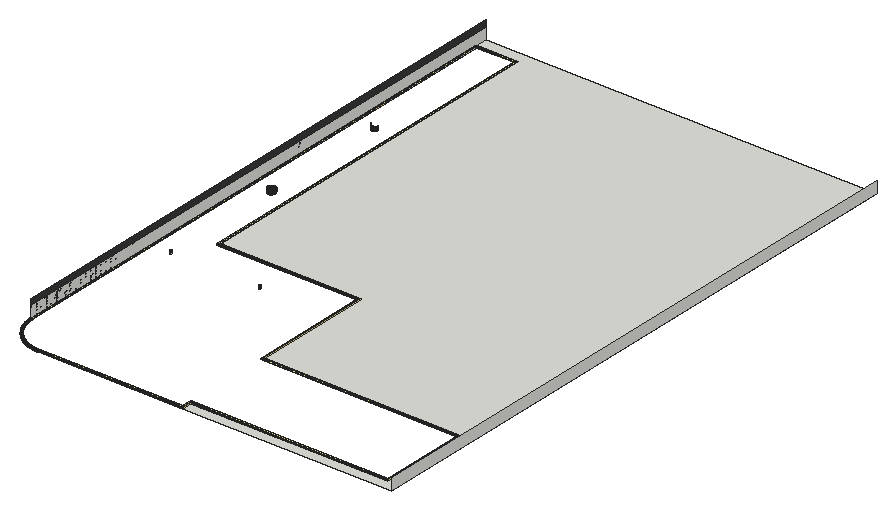
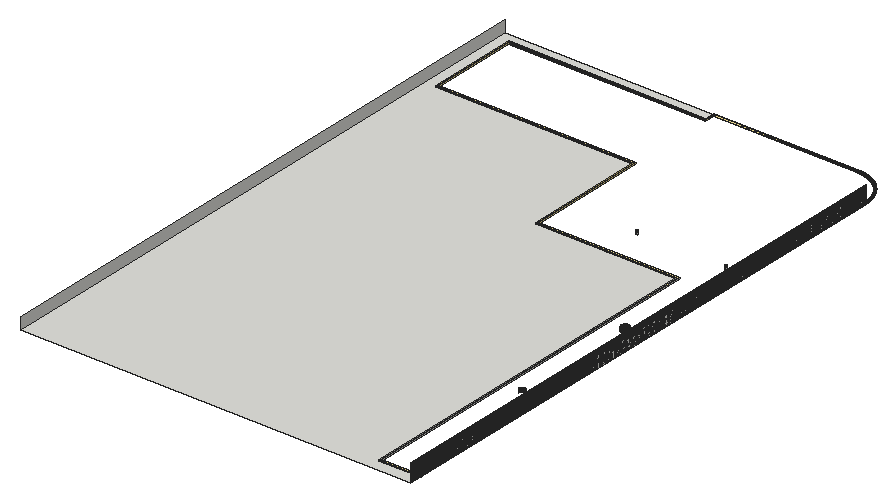
# SketchUp Ruby script. Lengths in inches.
U = 1.inch
M = Sketchup.active_model
def pt(a) = Geom::Point3d.new(a.map { |v| v * U })
def face(e, loops, mat)
  f = e.add_face(loops[0].map { |a| pt(a) })
  loops[1..].each { |l| e.add_face(l.map { |a| pt(a) }).erase! }
  f.material = f.back_material = mat if mat
  f
end
# faces: each face lists its corners as indices into pts; further lists are holes
def faces(e, pts, list, mat = nil) = list.each { |f| face(e, (f[0].is_a?(Array) ? f : [f]).map { |l| l.map { |i| pts[i] } }, mat) }
# xy, xz, yz: faces in a plane at the given z, y or x. An outline is a flat list of corners, or four numbers for a rectangle; further outlines are holes
def ring(l) = l.size == 4 ? [[l[0], l[1]], [l[2], l[1]], [l[2], l[3]], [l[0], l[3]]] : l.each_slice(2).to_a
def flat(e, list, mat, &to3) = list.each { |f| face(e, (f[0].is_a?(Array) ? f : [f]).map { |l| ring(l).map { |u, v| to3.(u, v) } }, mat) }
def xy(e, z, list, mat = nil) = flat(e, list, mat) { |x, y| [x, y, z] }
def xz(e, y, list, mat = nil) = flat(e, list, mat) { |x, z| [x, y, z] }
def yz(e, x, list, mat = nil) = flat(e, list, mat) { |y, z| [x, y, z] }
def lines(e, pts, list) = list.each { |a, b| e.add_line(pt(pts[a]), pt(pts[b])) }
# prism: a flat outline (further loops are holes) pulled along v
def prism(e, loops, v, mat = nil)
  f = face(e, loops, mat); d = Geom::Vector3d.new(v.map { |x| x * U })
  f.pushpull(f.normal.samedirection?(d) ? d.length : -d.length)
end
def box(e, o, s, mat = nil) = prism(e, [[o, [o[0] + s[0], o[1], o[2]], [o[0] + s[0], o[1] + s[1], o[2]], [o[0], o[1] + s[1], o[2]]]], [0, 0, s[2]], mat)
def at(x, y, z, deg = 0) = Geom::Transformation.translation(pt([x, y, z])) * Geom::Transformation.rotation(ORIGIN, Z_AXIS, deg.degrees)
def axes(o, x, y, z) = Geom::Transformation.new([*x, 0, *y, 0, *z, 0, *pt(o).to_a, 1])
def part(name) = M.definitions.add(name)
# library, detail: a bought-in or finely detailed component or shape, given as its bounding box
def library(name, o, s) = part(name).tap { |d| box(d.entities, o, s) }
def detail(e, o, s) = box(e.add_group.entities, o, s)
def put(e, d, t, mat = nil) = e.add_instance(d, t).tap { |i| i.material = mat if mat }
def group(e, t, mat = nil) = e.add_group.tap { |g| g.transformation = t; g.material = mat if mat }.entities
root = M.entities
M.materials.add("1496 AP 8293 CARBON COPY").color = [58, 58, 58]
M.materials.add("False Ceiling Light").color = [251, 231, 149]
xy(root,129,[[158,85,158,93,314,93,314,165,158,165,158,261,47,261,47,555,14,555,14,564,323,564,323,85]])
xz(root,232.5,[[30.34,129,30.42,132],[30.42,129,30.5,132],[30.5,129,30.58,132],[30.58,129,30.66,132],[100.84,129,100.92,132],
  [100.92,129,101,132],[101,129,101.08,132],[101.08,129,101.16,132]])
xz(root,259.5,[[45.5,129,156.5,129.5]])
xz(root,261,[[47,129,158,129.5]])
xz(root,329,[[30.34,129,30.42,132],[30.42,129,30.5,132],[30.5,129,30.58,132],[30.58,129,30.66,132]])
xz(root,335,[[30.34,129,30.42,132],[30.42,129,30.5,132],[30.5,129,30.58,132],[30.58,129,30.66,132]])
xz(root,431.5,[[30.34,129,30.42,132],[30.42,129,30.5,132],[30.5,129,30.58,132],[30.58,129,30.66,132]])
yz(root,14,[[555,129,555,129.5,115,129.5,115,138,564,138,564,129]])
yz(root,14,[[115,129,564,143]],"1496 AP 8293 CARBON COPY")
yz(root,15.5,[[115,129,553.5,129.5]])
yz(root,27.5,[[331.84,129,331.92,132],[331.92,129,332,132],[332,129,332.08,132],[332.08,129,332.16,132]])
yz(root,33.5,[[331.84,129,331.92,132],[331.92,129,332,132],[332,129,332.08,132],[332.08,129,332.16,132]])
yz(root,45.5,[[259.5,129,553.5,129.5]])
yz(root,47,[[261,129,555,129.5]])
yz(root,323,[[85,129,564,138]])
p = [[30.97,232.46,129],[31.05,232.45,129],[31.05,232.45,132],[30.97,232.46,132],[30.03,232.46,129],[30.11,232.47,129],
  [30.11,232.47,132],[30.03,232.46,132],[30.1875,232.48,129],[30.1875,232.48,132],[30.26,232.49,129],[30.26,232.49,132],
  [30.34,232.5,129],[30.34,232.5,132],[30.74,232.49,129],[30.8125,232.48,129],[30.8125,232.48,132],[30.74,232.49,132],
  [30.66,232.5,129],[30.66,232.5,132],[30.89,232.47,129],[30.89,232.47,132],[100.53,232.46,129],[100.61,232.47,129],
  [100.61,232.47,132],[100.53,232.46,132],[100.6875,232.48,129],[100.6875,232.48,132],[100.76,232.49,129],[100.76,232.49,132],
  [100.84,232.5,129],[100.84,232.5,132],[101.24,232.49,129],[101.3125,232.48,129],[101.3125,232.48,132],[101.24,232.49,132],
  [101.16,232.5,129],[101.16,232.5,132],[101.39,232.47,129],[101.39,232.47,132],[101.47,232.46,129],[101.47,232.46,132],
  [30.11,329.03,129],[30.03,329.04,129],[30.03,329.04,132],[30.11,329.03,132],[29.95,329.05,129],[29.95,329.05,132],
  [30.1875,329.02,129],[30.1875,329.02,132],[30.26,329.01,129],[30.26,329.01,132],[30.34,329,129],[30.34,329,132],
  [30.74,329.01,129],[30.66,329,129],[30.66,329,132],[30.74,329.01,132],[30.8125,329.02,129],[30.8125,329.02,132],
  [30.89,329.03,129],[30.89,329.03,132],[30.97,329.04,129],[30.97,329.04,132],[31.05,329.05,129],[31.05,329.05,132],
  [29.57,329.15,129],[29.5,329.17,129],[29.5,329.17,132],[29.57,329.15,132],[29.72,329.1,129],[29.65,329.125,129],
  [29.65,329.125,132],[29.72,329.1,132],[29.8,329.08,129],[29.8,329.08,132],[29.875,329.07,129],[29.875,329.07,132],
  [31.125,329.07,129],[31.125,329.07,132],[31.2,329.08,129],[31.2,329.08,132],[31.28,329.1,129],[31.28,329.1,132],
  [31.35,329.125,129],[31.35,329.125,132],[31.43,329.15,129],[31.43,329.15,132],[31.5,329.17,129],[31.5,329.17,132],
  [29.35,329.23,129],[29.28,329.26,129],[29.28,329.26,132],[29.35,329.23,132],[29.42,329.2,129],[29.42,329.2,132],
  [31.58,329.2,129],[31.58,329.2,132],[31.65,329.23,129],[31.65,329.23,132],[31.72,329.26,129],[31.72,329.26,132],
  [29.21,329.29,129],[29.14,329.33,129],[29.14,329.33,132],[29.21,329.29,132],[29.07,329.36,129],[29.07,329.36,132],
  [31.79,329.29,129],[31.79,329.29,132],[31.86,329.33,129],[31.86,329.33,132],[31.93,329.36,129],[31.93,329.36,132],
  [29,329.4,129],[28.93,329.44,129],[28.93,329.44,132],[29,329.4,132],[28.87,329.48,129],[28.87,329.48,132],
  [32,329.4,129],[32,329.4,132],[32.07,329.44,129],[32.07,329.44,132],[32.13,329.48,129],[32.13,329.48,132],
  [28.8,329.53,129],[28.74,329.57,129],[28.74,329.57,132],[28.8,329.53,132],[32.2,329.53,129],[32.2,329.53,132],
  [32.26,329.57,129],[32.26,329.57,132],[28.67,329.62,129],[28.61,329.67,129],[28.61,329.67,132],[28.67,329.62,132],
  [32.33,329.62,129],[32.33,329.62,132],[32.39,329.67,129],[32.39,329.67,132],[28.55,329.72,129],[28.49,329.77,129],
  [28.49,329.77,132],[28.55,329.72,132],[32.45,329.72,129],[32.45,329.72,132],[32.51,329.77,129],[32.51,329.77,132],
  [28.43,329.82,129],[28.43,329.82,132],[28.38,329.88,129],[28.38,329.88,132],[32.57,329.82,129],[32.57,329.82,132],
  [32.62,329.88,129],[32.62,329.88,132],[28.32,329.93,129],[28.32,329.93,132],[28.27,329.99,129],[28.27,329.99,132],
  [32.68,329.93,129],[32.68,329.93,132],[32.73,329.99,129],[32.73,329.99,132],[28.22,330.05,129],[28.22,330.05,132],
  [32.78,330.05,129],[32.78,330.05,132],[28.17,330.11,129],[28.12,330.17,129],[28.12,330.17,132],[28.17,330.11,132],
  [32.83,330.11,129],[32.83,330.11,132],[32.88,330.17,129],[32.88,330.17,132],[28.07,330.24,129],[28.03,330.3,129],
  [28.03,330.3,132],[28.07,330.24,132],[32.93,330.24,129],[32.93,330.24,132],[32.97,330.3,129],[32.97,330.3,132],
  [27.98,330.37,129],[27.98,330.37,132],[33.02,330.37,129],[33.02,330.37,132],[27.94,330.43,129],[27.94,330.43,132],
  [27.9,330.5,129],[27.9,330.5,132],[33.06,330.43,129],[33.06,330.43,132],[33.1,330.5,129],[33.1,330.5,132],
  [27.86,330.57,129],[27.86,330.57,132],[33.14,330.57,129],[33.14,330.57,132],[27.83,330.64,129],[27.83,330.64,132],
  [27.79,330.71,129],[27.79,330.71,132],[33.17,330.64,129],[33.17,330.64,132],[33.21,330.71,129],[33.21,330.71,132],
  [27.76,330.78,129],[27.76,330.78,132],[33.24,330.78,129],[33.24,330.78,132],[27.73,330.85,129],[27.73,330.85,132],
  [33.27,330.85,129],[33.27,330.85,132],[27.7,330.92,129],[27.7,330.92,132],[27.67,331,129],[27.67,331,132],
  [33.3,330.92,129],[33.3,330.92,132],[33.33,331,129],[33.33,331,132],[27.65,331.07,129],[27.65,331.07,132],
  [33.35,331.07,129],[33.35,331.07,132],[27.625,331.15,129],[27.625,331.15,132],[27.6,331.22,129],[27.6,331.22,132],
  [33.375,331.15,129],[33.375,331.15,132],[33.4,331.22,129],[33.4,331.22,132],[27.58,331.3,129],[27.58,331.3,132],
  [33.42,331.3,129],[33.42,331.3,132],[27.57,331.375,129],[27.57,331.375,132],[33.43,331.375,129],[33.43,331.375,132],
  [27.55,331.45,129],[27.55,331.45,132],[33.45,331.45,129],[33.45,331.45,132],[27.54,331.53,129],[27.54,331.53,132],
  [27.53,331.61,129],[27.53,331.61,132],[33.46,331.53,129],[33.46,331.53,132],[33.47,331.61,129],[33.47,331.61,132],
  [27.52,331.6875,129],[27.52,331.6875,132],[33.48,331.6875,129],[33.48,331.6875,132],[27.51,331.76,129],[27.51,331.76,132],
  [33.49,331.76,129],[33.49,331.76,132],[27.5,331.84,129],[27.5,331.84,132],[33.5,331.84,129],[33.5,331.84,132],
  [27.5,332.16,129],[27.51,332.24,129],[27.51,332.24,132],[27.5,332.16,132],[27.52,332.3125,129],[27.52,332.3125,132],
  [33.49,332.24,129],[33.5,332.16,129],[33.5,332.16,132],[33.49,332.24,132],[33.48,332.3125,129],[33.48,332.3125,132],
  [27.53,332.39,129],[27.53,332.39,132],[33.47,332.39,129],[33.47,332.39,132],[27.54,332.47,129],[27.54,332.47,132],
  [33.46,332.47,129],[33.46,332.47,132],[27.55,332.55,129],[27.55,332.55,132],[27.57,332.625,129],[27.57,332.625,132],
  [33.45,332.55,129],[33.45,332.55,132],[33.43,332.625,129],[33.43,332.625,132],[27.58,332.7,129],[27.58,332.7,132],
  [33.42,332.7,129],[33.42,332.7,132],[27.6,332.78,129],[27.6,332.78,132],[33.4,332.78,129],[33.4,332.78,132],
  [27.625,332.85,129],[27.625,332.85,132],[33.375,332.85,129],[33.375,332.85,132],[27.65,332.93,129],[27.65,332.93,132],
  [27.67,333,129],[27.67,333,132],[33.33,333,129],[33.35,332.93,129],[33.35,332.93,132],[33.33,333,132],
  [27.7,333.08,129],[27.7,333.08,132],[33.3,333.08,129],[33.3,333.08,132],[27.73,333.15,129],[27.73,333.15,132],
  [27.76,333.22,129],[27.76,333.22,132],[33.24,333.22,129],[33.27,333.15,129],[33.27,333.15,132],[33.24,333.22,132],
  [27.79,333.29,129],[27.79,333.29,132],[33.21,333.29,129],[33.21,333.29,132],[27.83,333.36,129],[27.83,333.36,132],
  [33.17,333.36,129],[33.17,333.36,132],[27.86,333.43,129],[27.86,333.43,132],[27.9,333.5,129],[27.9,333.5,132],
  [33.14,333.43,129],[33.14,333.43,132],[33.1,333.5,129],[33.1,333.5,132],[27.94,333.57,129],[27.94,333.57,132],
  [33.06,333.57,129],[33.06,333.57,132],[27.98,333.63,129],[27.98,333.63,132],[28.03,333.7,129],[28.03,333.7,132],
  [33.02,333.63,129],[33.02,333.63,132],[32.97,333.7,129],[32.97,333.7,132],[28.07,333.76,129],[28.07,333.76,132],
  [32.93,333.76,129],[32.93,333.76,132],[28.12,333.83,129],[28.12,333.83,132],[28.17,333.89,129],[28.17,333.89,132],
  [32.83,333.89,129],[32.88,333.83,129],[32.88,333.83,132],[32.83,333.89,132],[28.22,333.95,129],[28.22,333.95,132],
  [28.27,334.01,129],[28.27,334.01,132],[32.73,334.01,129],[32.78,333.95,129],[32.78,333.95,132],[32.73,334.01,132],
  [28.32,334.07,129],[28.32,334.07,132],[32.68,334.07,129],[32.68,334.07,132],[28.38,334.12,129],[28.38,334.12,132],
  [28.43,334.18,129],[28.43,334.18,132],[32.62,334.12,129],[32.62,334.12,132],[32.57,334.18,129],[32.57,334.18,132],
  [28.49,334.23,129],[28.49,334.23,132],[28.55,334.28,129],[28.55,334.28,132],[32.45,334.28,129],[32.51,334.23,129],
  [32.51,334.23,132],[32.45,334.28,132],[28.61,334.33,129],[28.61,334.33,132],[28.67,334.38,129],[28.67,334.38,132],
  [32.33,334.38,129],[32.39,334.33,129],[32.39,334.33,132],[32.33,334.38,132],[28.74,334.43,129],[28.74,334.43,132],
  [28.8,334.47,129],[28.8,334.47,132],[32.2,334.47,129],[32.26,334.43,129],[32.26,334.43,132],[32.2,334.47,132],
  [28.87,334.52,129],[28.87,334.52,132],[28.93,334.56,129],[28.93,334.56,132],[32.13,334.52,129],[32.13,334.52,132],
  [32.07,334.56,129],[32.07,334.56,132],[29,334.6,129],[29,334.6,132],[29.07,334.64,129],[29.07,334.64,132],
  [29.14,334.67,129],[29.14,334.67,132],[31.93,334.64,129],[32,334.6,129],[32,334.6,132],[31.93,334.64,132],
  [31.86,334.67,129],[31.86,334.67,132],[29.21,334.71,129],[29.21,334.71,132],[29.28,334.74,129],[29.28,334.74,132],
  [29.35,334.77,129],[29.35,334.77,132],[31.65,334.77,129],[31.72,334.74,129],[31.72,334.74,132],[31.65,334.77,132],
  [31.79,334.71,129],[31.79,334.71,132],[29.42,334.8,129],[29.42,334.8,132],[29.5,334.83,129],[29.5,334.83,132],
  [29.57,334.85,129],[29.57,334.85,132],[31.43,334.85,129],[31.5,334.83,129],[31.5,334.83,132],[31.43,334.85,132],
  [31.58,334.8,129],[31.58,334.8,132],[29.65,334.875,129],[29.65,334.875,132],[29.72,334.9,129],[29.72,334.9,132],
  [29.8,334.92,129],[29.8,334.92,132],[29.875,334.93,129],[29.875,334.93,132],[29.95,334.95,129],[29.95,334.95,132],
  [30.03,334.96,129],[30.03,334.96,132],[31.05,334.95,129],[31.125,334.93,129],[31.125,334.93,132],[31.05,334.95,132],
  [30.97,334.96,129],[30.97,334.96,132],[31.2,334.92,129],[31.2,334.92,132],[31.28,334.9,129],[31.28,334.9,132],
  [31.35,334.875,129],[31.35,334.875,132],[30.11,334.97,129],[30.11,334.97,132],[30.1875,334.98,129],[30.1875,334.98,132],
  [30.26,334.99,129],[30.26,334.99,132],[30.34,335,129],[30.34,335,132],[30.74,334.99,129],[30.8125,334.98,129],
  [30.8125,334.98,132],[30.74,334.99,132],[30.66,335,129],[30.66,335,132],[30.89,334.97,129],[30.89,334.97,132],
  [30.11,431.53,129],[30.03,431.54,129],[30.03,431.54,132],[30.11,431.53,132],[29.95,431.55,129],[29.95,431.55,132],
  [30.1875,431.52,129],[30.1875,431.52,132],[30.26,431.51,129],[30.26,431.51,132],[30.34,431.5,129],[30.34,431.5,132],
  [30.74,431.51,129],[30.66,431.5,129],[30.66,431.5,132],[30.74,431.51,132],[30.8125,431.52,129],[30.8125,431.52,132],
  [30.89,431.53,129],[30.89,431.53,132],[30.97,431.54,129],[30.97,431.54,132],[31.05,431.55,129],[31.05,431.55,132],
  [29.57,431.65,129],[29.5,431.67,129],[29.5,431.67,132],[29.57,431.65,132],[29.72,431.6,129],[29.65,431.625,129],
  [29.65,431.625,132],[29.72,431.6,132],[29.8,431.58,129],[29.8,431.58,132],[29.875,431.57,129],[29.875,431.57,132],
  [31.125,431.57,129],[31.125,431.57,132],[31.2,431.58,129],[31.2,431.58,132],[31.28,431.6,129],[31.28,431.6,132],
  [31.35,431.625,129],[31.35,431.625,132],[31.43,431.65,129],[31.43,431.65,132],[31.5,431.67,129],[31.5,431.67,132],
  [29.35,431.73,129],[29.28,431.76,129],[29.28,431.76,132],[29.35,431.73,132],[29.42,431.7,129],[29.42,431.7,132],
  [31.58,431.7,129],[31.58,431.7,132],[31.65,431.73,129],[31.65,431.73,132],[31.72,431.76,129],[31.72,431.76,132],
  [29.21,431.79,129],[29.14,431.83,129],[29.14,431.83,132],[29.21,431.79,132],[29.07,431.86,129],[29.07,431.86,132],
  [31.79,431.79,129],[31.79,431.79,132],[31.86,431.83,129],[31.86,431.83,132],[31.93,431.86,129],[31.93,431.86,132],
  [29,431.9,129],[28.93,431.94,129],[28.93,431.94,132],[29,431.9,132],[28.87,431.98,129],[28.87,431.98,132],
  [32,431.9,129],[32,431.9,132],[32.07,431.94,129],[32.07,431.94,132],[32.13,431.98,129],[32.13,431.98,132],
  [28.8,432.03,129],[28.74,432.07,129],[28.74,432.07,132],[28.8,432.03,132],[32.2,432.03,129],[32.2,432.03,132],
  [32.26,432.07,129],[32.26,432.07,132],[28.67,432.12,129],[28.61,432.17,129],[28.61,432.17,132],[28.67,432.12,132],
  [32.33,432.12,129],[32.33,432.12,132],[32.39,432.17,129],[32.39,432.17,132],[28.55,432.22,129],[28.49,432.27,129],
  [28.49,432.27,132],[28.55,432.22,132],[32.45,432.22,129],[32.45,432.22,132],[32.51,432.27,129],[32.51,432.27,132],
  [28.43,432.32,129],[28.43,432.32,132],[28.38,432.38,129],[28.38,432.38,132],[32.57,432.32,129],[32.57,432.32,132],
  [32.62,432.38,129],[32.62,432.38,132],[28.32,432.43,129],[28.32,432.43,132],[28.27,432.49,129],[28.27,432.49,132],
  [32.68,432.43,129],[32.68,432.43,132],[32.73,432.49,129],[32.73,432.49,132],[28.22,432.55,129],[28.22,432.55,132],
  [32.78,432.55,129],[32.78,432.55,132],[28.17,432.61,129],[28.12,432.67,129],[28.12,432.67,132],[28.17,432.61,132],
  [32.83,432.61,129],[32.83,432.61,132],[32.88,432.67,129],[32.88,432.67,132],[28.07,432.74,129],[28.03,432.8,129],
  [28.03,432.8,132],[28.07,432.74,132],[32.93,432.74,129],[32.93,432.74,132],[32.97,432.8,129],[32.97,432.8,132],
  [27.98,432.87,129],[27.98,432.87,132],[33.02,432.87,129],[33.02,432.87,132],[27.94,432.93,129],[27.94,432.93,132],
  [27.9,433,129],[27.9,433,132],[33.06,432.93,129],[33.06,432.93,132],[33.1,433,129],[33.1,433,132],
  [27.86,433.07,129],[27.86,433.07,132],[33.14,433.07,129],[33.14,433.07,132],[27.83,433.14,129],[27.83,433.14,132],
  [27.79,433.21,129],[27.79,433.21,132],[33.17,433.14,129],[33.17,433.14,132],[33.21,433.21,129],[33.21,433.21,132],
  [27.76,433.28,129],[27.76,433.28,132],[33.24,433.28,129],[33.24,433.28,132],[27.73,433.35,129],[27.73,433.35,132],
  [33.27,433.35,129],[33.27,433.35,132],[27.7,433.42,129],[27.7,433.42,132],[27.67,433.5,129],[27.67,433.5,132],
  [33.3,433.42,129],[33.3,433.42,132],[33.33,433.5,129],[33.33,433.5,132],[27.65,433.57,129],[27.65,433.57,132],
  [33.35,433.57,129],[33.35,433.57,132],[27.625,433.65,129],[27.625,433.65,132],[27.6,433.72,129],[27.6,433.72,132],
  [33.375,433.65,129],[33.375,433.65,132],[33.4,433.72,129],[33.4,433.72,132],[27.58,433.8,129],[27.58,433.8,132],
  [33.42,433.8,129],[33.42,433.8,132],[27.57,433.875,129],[27.57,433.875,132],[33.43,433.875,129],[33.43,433.875,132]]
faces(root,p,[[0,1,2,3],[4,5,6,7],[5,8,9,6],[8,10,11,9],[10,12,13,11],[14,15,16,17],[18,14,17,19],[15,20,21,16],
  [20,0,3,21],[22,23,24,25],[23,26,27,24],[26,28,29,27],[28,30,31,29],[32,33,34,35],[36,32,35,37],[33,38,39,34],
  [38,40,41,39],[42,43,44,45],[43,46,47,44],[48,42,45,49],[50,48,49,51],[52,50,51,53],[54,55,56,57],[58,54,57,59],
  [60,58,59,61],[62,60,61,63],[64,62,63,65],[66,67,68,69],[70,71,72,73],[71,66,69,72],[74,70,73,75],[76,74,75,77],
  [46,76,77,47],[78,64,65,79],[80,78,79,81],[82,80,81,83],[84,82,83,85],[86,84,85,87],[88,86,87,89],[90,91,92,93],
  [67,94,95,68],[94,90,93,95],[96,88,89,97],[98,96,97,99],[100,98,99,101],[102,103,104,105],[103,106,107,104],[91,102,105,92],
  [108,100,101,109],[110,108,109,111],[112,110,111,113],[114,115,116,117],[115,118,119,116],[106,114,117,107],[120,112,113,121],[122,120,121,123],
  [124,122,123,125],[126,127,128,129],[118,126,129,119],[130,124,125,131],[132,130,131,133],[134,135,136,137],[127,134,137,128],[138,132,133,139],
  [140,138,139,141],[142,143,144,145],[135,142,145,136],[146,140,141,147],[148,146,147,149],[143,150,151,144],[150,152,153,151],[154,148,149,155],
  [156,154,155,157],[152,158,159,153],[158,160,161,159],[162,156,157,163],[164,162,163,165],[160,166,167,161],[168,164,165,169],[170,171,172,173],
  [166,170,173,167],[174,168,169,175],[176,174,175,177],[178,179,180,181],[171,178,181,172],[182,176,177,183],[184,182,183,185],[179,186,187,180],
  [188,184,185,189],[186,190,191,187],[190,192,193,191],[194,188,189,195],[196,194,195,197],[192,198,199,193],[200,196,197,201],[198,202,203,199],
  [202,204,205,203],[206,200,201,207],[208,206,207,209],[204,210,211,205],[212,208,209,213],[210,214,215,211],[216,212,213,217],[214,218,219,215],
  [218,220,221,219],[222,216,217,223],[224,222,223,225],[220,226,227,221],[228,224,225,229],[226,230,231,227],[230,232,233,231],[234,228,229,235],
  [236,234,235,237],[232,238,239,233],[240,236,237,241],[238,242,243,239],[244,240,241,245],[242,246,247,243],[248,244,245,249],[246,250,251,247],
  [250,252,253,251],[254,248,249,255],[256,254,255,257],[252,258,259,253],[260,256,257,261],[258,262,263,259],[264,260,261,265],[262,266,267,263],
  [268,264,265,269],[270,271,272,273],[271,274,275,272],[276,277,278,279],[280,276,279,281],[274,282,283,275],[284,280,281,285],[282,286,287,283],
  [288,284,285,289],[286,290,291,287],[290,292,293,291],[294,288,289,295],[296,294,295,297],[292,298,299,293],[300,296,297,301],[298,302,303,299],
  [304,300,301,305],[302,306,307,303],[308,304,305,309],[306,310,311,307],[310,312,313,311],[314,315,316,317],[315,308,309,316],[312,318,319,313],
  [320,314,317,321],[318,322,323,319],[322,324,325,323],[326,327,328,329],[327,320,321,328],[324,330,331,325],[332,326,329,333],[330,334,335,331],
  [336,332,333,337],[334,338,339,335],[338,340,341,339],[342,336,337,343],[344,342,343,345],[340,346,347,341],[348,344,345,349],[346,350,351,347],
  [350,352,353,351],[354,348,349,355],[356,354,355,357],[352,358,359,353],[360,356,357,361],[358,362,363,359],[362,364,365,363],[366,367,368,369],
  [367,360,361,368],[364,370,371,365],[370,372,373,371],[374,375,376,377],[375,366,369,376],[372,378,379,373],[380,374,377,381],[378,382,383,379],
  [382,384,385,383],[386,380,381,387],[388,386,387,389],[384,390,391,385],[390,392,393,391],[394,395,396,397],[395,388,389,396],[392,398,399,393],
  [398,400,401,399],[402,403,404,405],[403,394,397,404],[400,406,407,401],[406,408,409,407],[410,411,412,413],[411,402,405,412],[408,414,415,409],
  [414,416,417,415],[418,410,413,419],[420,418,419,421],[416,422,423,417],[422,424,425,423],[424,426,427,425],[428,429,430,431],[432,428,431,433],
  [429,420,421,430],[426,434,435,427],[434,436,437,435],[436,438,439,437],[440,441,442,443],[441,444,445,442],[444,432,433,445],[438,446,447,439],
  [446,448,449,447],[448,450,451,449],[452,453,454,455],[453,456,457,454],[456,440,443,457],[450,458,459,451],[458,460,461,459],[460,462,463,461],
  [462,464,465,463],[464,466,467,465],[466,468,469,467],[470,471,472,473],[474,470,473,475],[471,476,477,472],[476,478,479,477],[478,480,481,479],
  [480,452,455,481],[468,482,483,469],[482,484,485,483],[484,486,487,485],[486,488,489,487],[490,491,492,493],[494,490,493,495],[491,496,497,492],
  [496,474,475,497],[498,499,500,501],[499,502,503,500],[504,498,501,505],[506,504,505,507],[508,506,507,509],[510,511,512,513],[514,510,513,515],
  [516,514,515,517],[518,516,517,519],[520,518,519,521],[522,523,524,525],[526,527,528,529],[527,522,525,528],[530,526,529,531],[532,530,531,533],
  [502,532,533,503],[534,520,521,535],[536,534,535,537],[538,536,537,539],[540,538,539,541],[542,540,541,543],[544,542,543,545],[546,547,548,549],
  [523,550,551,524],[550,546,549,551],[552,544,545,553],[554,552,553,555],[556,554,555,557],[558,559,560,561],[559,562,563,560],[547,558,561,548],
  [564,556,557,565],[566,564,565,567],[568,566,567,569],[570,571,572,573],[571,574,575,572],[562,570,573,563],[576,568,569,577],[578,576,577,579],
  [580,578,579,581],[582,583,584,585],[574,582,585,575],[586,580,581,587],[588,586,587,589],[590,591,592,593],[583,590,593,584],[594,588,589,595],
  [596,594,595,597],[598,599,600,601],[591,598,601,592],[602,596,597,603],[604,602,603,605],[599,606,607,600],[606,608,609,607],[610,604,605,611],
  [612,610,611,613],[608,614,615,609],[614,616,617,615],[618,612,613,619],[620,618,619,621],[616,622,623,617],[624,620,621,625],[626,627,628,629],
  [622,626,629,623],[630,624,625,631],[632,630,631,633],[634,635,636,637],[627,634,637,628],[638,632,633,639],[640,638,639,641],[635,642,643,636],
  [644,640,641,645],[642,646,647,643],[646,648,649,647],[650,644,645,651],[652,650,651,653],[648,654,655,649],[656,652,653,657],[654,658,659,655],
  [658,660,661,659],[662,656,657,663],[664,662,663,665],[660,666,667,661],[668,664,665,669],[666,670,671,667],[672,668,669,673],[670,674,675,671],
  [674,676,677,675],[678,672,673,679],[680,678,679,681],[676,682,683,677],[684,680,681,685],[682,686,687,683],[686,688,689,687],[690,684,685,691],
  [692,690,691,693],[688,694,695,689],[696,692,693,697],[694,698,699,695],[700,696,697,701]])
g1 = group(root,at(14,85,129),"False Ceiling Light")
prism(g1,[[[0,30,0],[0,470,0],[33,470,0],[33,176,0],[144,176,0],[144,80,0],[300,80,0],[300,8,0],[144,8,0],[144,0,0],[30,0,0],[29.61,0,0],[29.21,0.01,0],[28.82,0.02,0],[28.43,0.04,0],[28.04,0.0625,0],[27.65,0.09,0],[27.25,0.125,0],[26.86,0.16,0],[26.47,0.21,0],[26.08,0.26,0],[25.7,0.31,0],[25.31,0.37,0],[24.92,0.43,0],[24.53,0.5,0],[24.15,0.58,0],[23.76,0.66,0],[23.38,0.74,0],[23,0.83,0],[22.62,0.92,0],[22.24,1.02,0],[21.86,1.125,0],[21.48,1.24,0],[21.1,1.35,0],[20.73,1.47,0],[20.36,1.59,0],[19.99,1.72,0],[19.62,1.85,0],[19.25,1.99,0],[18.88,2.14,0],[18.52,2.28,0],[18.16,2.4375,0],[17.8,2.59,0],[17.44,2.76,0],[17.08,2.92,0],[16.73,3.09,0],[16.38,3.27,0],[16.03,3.45,0],[15.69,3.64,0],[15.34,3.83,0],[15,4.02,0],[14.66,4.22,0],[14.33,4.42,0],[13.99,4.63,0],[13.66,4.84,0],[13.33,5.06,0],[13.01,5.28,0],[12.6875,5.5,0],[12.37,5.73,0],[12.05,5.96,0],[11.74,6.2,0],[11.43,6.44,0],[11.12,6.6875,0],[10.82,6.93,0],[10.52,7.1875,0],[10.22,7.44,0],[9.93,7.71,0],[9.64,7.97,0],[9.35,8.24,0],[9.07,8.51,0],[8.79,8.79,0],[8.51,9.07,0],[8.24,9.35,0],[7.97,9.64,0],[7.71,9.93,0],[7.44,10.22,0],[7.1875,10.52,0],[6.93,10.82,0],[6.6875,11.12,0],[6.44,11.43,0],[6.2,11.74,0],[5.96,12.05,0],[5.73,12.37,0],[5.5,12.6875,0],[5.28,13.01,0],[5.06,13.33,0],[4.84,13.66,0],[4.63,13.99,0],[4.42,14.33,0],[4.22,14.66,0],[4.02,15,0],[3.83,15.34,0],[3.64,15.69,0],[3.45,16.03,0],[3.27,16.38,0],[3.09,16.73,0],[2.92,17.08,0],[2.76,17.44,0],[2.59,17.8,0],[2.4375,18.16,0],[2.28,18.52,0],[2.14,18.88,0],[1.99,19.25,0],[1.85,19.62,0],[1.72,19.99,0],[1.59,20.36,0],[1.47,20.73,0],[1.35,21.1,0],[1.24,21.48,0],[1.125,21.86,0],[1.02,22.24,0],[0.92,22.62,0],[0.83,23,0],[0.74,23.38,0],[0.66,23.76,0],[0.58,24.15,0],[0.5,24.53,0],[0.43,24.92,0],[0.37,25.31,0],[0.31,25.7,0],[0.26,26.08,0],[0.21,26.47,0],[0.16,26.86,0],[0.125,27.25,0],[0.09,27.65,0],[0.0625,28.04,0],[0.04,28.43,0],[0.02,28.82,0],[0.01,29.21,0],[0,29.61,0]],[[31.5,468.5,0],[1.5,468.5,0],[1.5,30,0],[1.5,29.625,0],[1.51,29.25,0],[1.52,28.88,0],[1.54,28.51,0],[1.5625,28.14,0],[1.59,27.76,0],[1.62,27.39,0],[1.66,27.02,0],[1.7,26.65,0],[1.74,26.28,0],[1.79,25.91,0],[1.85,25.54,0],[1.91,25.17,0],[1.98,24.81,0],[2.05,24.44,0],[2.12,24.07,0],[2.2,23.71,0],[2.29,23.35,0],[2.375,22.98,0],[2.47,22.625,0],[2.57,22.26,0],[2.67,21.91,0],[2.78,21.55,0],[2.89,21.19,0],[3.01,20.84,0],[3.13,20.49,0],[3.26,20.14,0],[3.39,19.79,0],[3.53,19.4375,0],[3.67,19.09,0],[3.8125,18.75,0],[3.96,18.41,0],[4.12,18.07,0],[4.28,17.73,0],[4.4375,17.39,0],[4.61,17.0625,0],[4.78,16.73,0],[4.95,16.4,0],[5.13,16.07,0],[5.32,15.75,0],[5.51,15.43,0],[5.7,15.11,0],[5.9,14.79,0],[6.1,14.48,0],[6.3,14.17,0],[6.51,13.86,0],[6.73,13.55,0],[6.94,13.25,0],[7.16,12.95,0],[7.39,12.65,0],[7.62,12.36,0],[7.85,12.0625,0],[8.09,11.78,0],[8.33,11.49,0],[8.57,11.21,0],[8.82,10.93,0],[9.07,10.65,0],[9.33,10.38,0],[9.59,10.11,0],[9.85,9.85,0],[10.11,9.59,0],[10.38,9.33,0],[10.65,9.07,0],[10.93,8.82,0],[11.21,8.57,0],[11.49,8.33,0],[11.78,8.09,0],[12.0625,7.85,0],[12.36,7.62,0],[12.65,7.39,0],[12.95,7.16,0],[13.25,6.94,0],[13.55,6.73,0],[13.86,6.51,0],[14.17,6.3,0],[14.48,6.1,0],[14.79,5.9,0],[15.11,5.7,0],[15.43,5.51,0],[15.75,5.32,0],[16.07,5.13,0],[16.4,4.95,0],[16.73,4.78,0],[17.0625,4.61,0],[17.39,4.4375,0],[17.73,4.28,0],[18.07,4.12,0],[18.41,3.96,0],[18.75,3.8125,0],[19.09,3.67,0],[19.4375,3.53,0],[19.79,3.39,0],[20.14,3.26,0],[20.49,3.13,0],[20.84,3.01,0],[21.19,2.89,0],[21.55,2.78,0],[21.91,2.67,0],[22.26,2.57,0],[22.625,2.47,0],[22.98,2.375,0],[23.35,2.29,0],[23.71,2.2,0],[24.07,2.12,0],[24.44,2.05,0],[24.81,1.98,0],[25.17,1.91,0],[25.54,1.85,0],[25.91,1.79,0],[26.28,1.74,0],[26.65,1.7,0],[27.02,1.66,0],[27.39,1.62,0],[27.76,1.59,0],[28.14,1.5625,0],[28.51,1.54,0],[28.88,1.52,0],[29.25,1.51,0],[29.625,1.5,0],[30,1.5,0],[142.5,1.5,0],[142.5,9.5,0],[298.5,9.5,0],[298.5,78.5,0],[142.5,78.5,0],[142.5,174.5,0],[31.5,174.5,0]]],[0,0,0.5])
